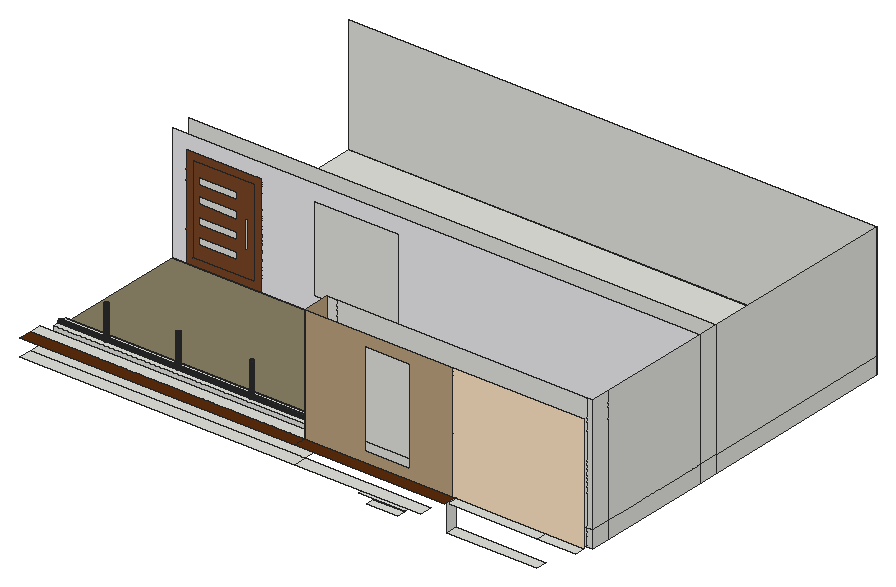
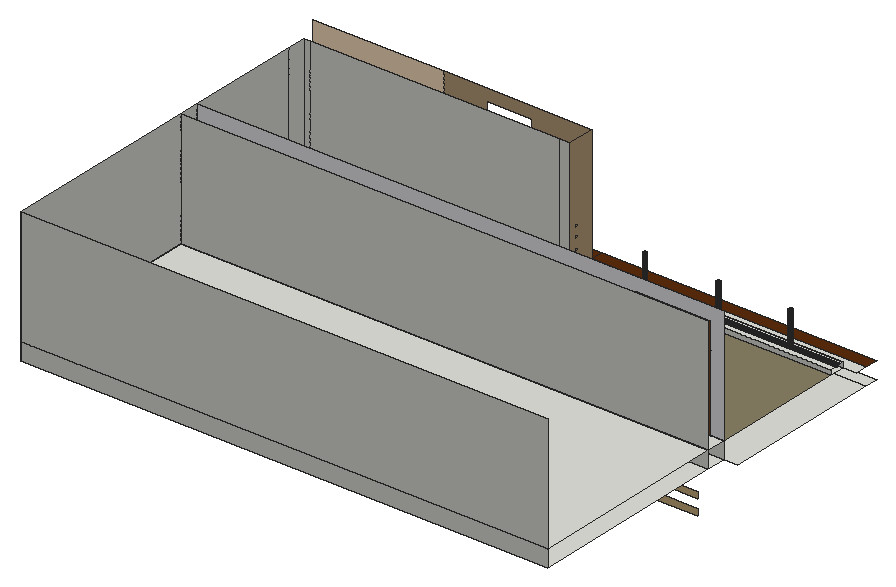
# SketchUp Ruby script. Lengths in inches.
U = 1.inch
M = Sketchup.active_model
def pt(a) = Geom::Point3d.new(a.map { |v| v * U })
def face(e, loops, mat)
  f = e.add_face(loops[0].map { |a| pt(a) })
  loops[1..].each { |l| e.add_face(l.map { |a| pt(a) }).erase! }
  f.material = f.back_material = mat if mat
  f
end
# faces: each face lists its corners as indices into pts; further lists are holes
def faces(e, pts, list, mat = nil) = list.each { |f| face(e, (f[0].is_a?(Array) ? f : [f]).map { |l| l.map { |i| pts[i] } }, mat) }
# xy, xz, yz: faces in a plane at the given z, y or x. An outline is a flat list of corners, or four numbers for a rectangle; further outlines are holes
def ring(l) = l.size == 4 ? [[l[0], l[1]], [l[2], l[1]], [l[2], l[3]], [l[0], l[3]]] : l.each_slice(2).to_a
def flat(e, list, mat, &to3) = list.each { |f| face(e, (f[0].is_a?(Array) ? f : [f]).map { |l| ring(l).map { |u, v| to3.(u, v) } }, mat) }
def xy(e, z, list, mat = nil) = flat(e, list, mat) { |x, y| [x, y, z] }
def xz(e, y, list, mat = nil) = flat(e, list, mat) { |x, z| [x, y, z] }
def yz(e, x, list, mat = nil) = flat(e, list, mat) { |y, z| [x, y, z] }
def lines(e, pts, list) = list.each { |a, b| e.add_line(pt(pts[a]), pt(pts[b])) }
# prism: a flat outline (further loops are holes) pulled along v
def prism(e, loops, v, mat = nil)
  f = face(e, loops, mat); d = Geom::Vector3d.new(v.map { |x| x * U })
  f.pushpull(f.normal.samedirection?(d) ? d.length : -d.length)
end
def box(e, o, s, mat = nil) = prism(e, [[o, [o[0] + s[0], o[1], o[2]], [o[0] + s[0], o[1] + s[1], o[2]], [o[0], o[1] + s[1], o[2]]]], [0, 0, s[2]], mat)
def at(x, y, z, deg = 0) = Geom::Transformation.translation(pt([x, y, z])) * Geom::Transformation.rotation(ORIGIN, Z_AXIS, deg.degrees)
def axes(o, x, y, z) = Geom::Transformation.new([*x, 0, *y, 0, *z, 0, *pt(o).to_a, 1])
def part(name) = M.definitions.add(name)
# library, detail: a bought-in or finely detailed component or shape, given as its bounding box
def library(name, o, s) = part(name).tap { |d| box(d.entities, o, s) }
def detail(e, o, s) = box(e.add_group.entities, o, s)
def put(e, d, t, mat = nil) = e.add_instance(d, t).tap { |i| i.material = mat if mat }
def group(e, t, mat = nil) = e.add_group.tap { |g| g.transformation = t; g.material = mat if mat }.entities
root = M.entities
M.materials.add("[0012_Bisque]").color = [255, 228, 196]
M.materials.add("[0035_Tan]").color = [188, 161, 125]
M.materials.add("[0043_SaddleBrown]").color = [91, 44, 12]
M.materials.add("[Blinds Vertical Pattern]").color = [237, 237, 239]
M.materials.add("[Carpet Pattern Squares Multi]").color = [138, 129, 101]
M.materials.add("[Color M07]").color = [58, 58, 58]
M.materials.add("[Formica Beige]").color = [211, 187, 149]
M.materials.add("[Wood Floor Light]").color = [204, 176, 127]
M.materials.add("[Wood Veneer 01]").color = [120, 70, 37]
xy(root,367.68,[[212.94,538.2,295.68,547.45]],"[Formica Beige]")
xy(root,369.94,[[382.27,385.97,410.625,393.34]])
xy(root,373.6,[[456.39,383.84,537.68,393.34]])
xy(root,376.36,[[375.85,385.97,417.04,393.34]])
xy(root,381.625,[[73.92,382.09,320.99,393.34],[320.99,382.09,434.25,393.34],[73.92,393.34,73.92,538.2,329.72,538.2,329.72,418.04,320.99,418.04,320.99,393.34],[329.72,418.04,560.26,538.2],[85.98,538.2,329.72,556.28],
  [329.72,538.2,560.26,556.28],[85.98,556.28,560.26,737.09]])
xy(root,397.0625,[[456.39,383.84,537.68,393.34],[537.68,383.84,572.32,393.34],[73.92,393.34,320.99,404.34],[[85.98,404.34,320.99,418.04],[128.47,408.87,128.9,408.93,129.31,409.1,129.66,409.36,129.93,409.71,130.1,410.12,130.15,410.56,130.1,410.99,129.93,411.4,129.66,411.75,129.31,412.02,128.9,412.1875,128.47,412.25,128.03,412.1875,127.62,412.02,127.27,411.75,127,411.4,126.84,410.99,126.78,410.56,126.84,410.12,127,409.71,127.27,409.36,127.62,409.1,128.03,408.93],[259.47,408.87,259.9,408.93,260.31,409.1,260.66,409.36,260.93,409.71,261.1,410.12,261.15,410.56,261.1,410.99,260.93,411.4,260.66,411.75,260.31,412.02,259.9,412.1875,259.47,412.25,259.03,412.1875,258.62,412.02,258.27,411.75,258,411.4,257.84,410.99,257.78,410.56,257.84,410.12,258,409.71,258.27,409.36,258.62,409.1,259.03,408.93],[193.34,408.87,193.78,408.93,194.18,409.1,194.53,409.36,194.8,409.71,194.97,410.12,195.03,410.56,194.97,410.99,194.8,411.4,194.53,411.75,194.18,412.02,193.78,412.1875,193.34,412.25,192.9,412.1875,192.5,412.02,192.15,411.75,191.88,411.4,191.71,410.99,191.65,410.56,191.71,410.12,191.88,409.71,192.15,409.36,192.5,409.1,192.9,408.93]],[128.47,408.87,128.03,408.93,127.62,409.1,127.27,409.36,127,409.71,126.84,410.12,126.78,410.56,126.84,410.99,127,411.4,127.27,411.75,127.62,412.02,128.03,412.1875,128.47,412.25,128.9,412.1875,129.31,412.02,129.66,411.75,129.93,411.4,130.1,410.99,130.15,410.56,130.1,410.12,129.93,409.71,129.66,409.36,129.31,409.1,128.9,408.93],
  [193.34,408.87,192.9,408.93,192.5,409.1,192.15,409.36,191.88,409.71,191.71,410.12,191.65,410.56,191.71,410.99,191.88,411.4,192.15,411.75,192.5,412.02,192.9,412.1875,193.34,412.25,193.78,412.1875,194.18,412.02,194.53,411.75,194.8,411.4,194.97,410.99,195.03,410.56,194.97,410.12,194.8,409.71,194.53,409.36,194.18,409.1,193.78,408.93],[259.47,408.87,259.03,408.93,258.62,409.1,258.27,409.36,258,409.71,257.84,410.12,257.78,410.56,257.84,410.99,258,411.4,258.27,411.75,258.62,412.02,259.03,412.1875,259.47,412.25,259.9,412.1875,260.31,412.02,260.66,411.75,260.93,411.4,261.1,410.99,261.15,410.56,261.1,410.12,260.93,409.71,260.66,409.36,260.31,409.1,259.9,408.93],[85.98,538.2,560.26,556.28],[85.98,556.28,560.26,737.09]])
xy(root,397.0625,[[73.92,382.09,320.99,393.34],[320.99,382.09,456.39,393.34]],"[0043_SaddleBrown]")
xy(root,397.0625,[[85.98,418.04,560.26,538.2]],"[Carpet Pattern Squares Multi]")
xy(root,401.4375,[[[85.98,404.34,320.99,418.04],[128.47,408.87,128.03,408.93,127.62,409.1,127.27,409.36,127,409.71,126.84,410.12,126.78,410.56,126.84,410.99,127,411.4,127.27,411.75,127.62,412.02,128.03,412.1875,128.47,412.25,128.9,412.1875,129.31,412.02,129.66,411.75,129.93,411.4,130.1,410.99,130.15,410.56,130.1,410.12,129.93,409.71,129.66,409.36,129.31,409.1,128.9,408.93],[259.47,408.87,259.03,408.93,258.62,409.1,258.27,409.36,258,409.71,257.84,410.12,257.78,410.56,257.84,410.99,258,411.4,258.27,411.75,258.62,412.02,259.03,412.1875,259.47,412.25,259.9,412.1875,260.31,412.02,260.66,411.75,260.93,411.4,261.1,410.99,261.15,410.56,261.1,410.12,260.93,409.71,260.66,409.36,260.31,409.1,259.9,408.93],[193.34,408.87,192.9,408.93,192.5,409.1,192.15,409.36,191.88,409.71,191.71,410.12,191.65,410.56,191.71,410.99,191.88,411.4,192.15,411.75,192.5,412.02,192.9,412.1875,193.34,412.25,193.78,412.1875,194.18,412.02,194.53,411.75,194.8,411.4,194.97,410.99,195.03,410.56,194.97,410.12,194.8,409.71,194.53,409.36,194.18,409.1,193.78,408.93]]])
xz(root,393.34,[[454.48,397.0625,572.32,501.625]],"[0012_Bisque]")
xz(root,393.34,[[[320.99,397.0625,454.48,501.625],[374.52,406.1,415.58,491.35]]],"[0035_Tan]")
xz(root,404.34,[[85.98,397.0625,320.99,401.4375]])
xz(root,418.04,[[320.99,381.625,329.72,397.0625],[329.72,381.625,554.62,397.0625],[554.62,381.625,560.26,397.0625],[85.98,397.0625,320.99,401.4375],[320.99,397.0625,329.72,501.625],
  [329.72,397.0625,554.62,501.625],[554.62,397.0625,560.26,501.625]])
xz(root,538.2,[[85.98,381.625,560.26,397.0625]])
xz(root,538.2,[[[85.98,397.0625,97.73,397.0625,97.73,489,166.42,489,166.42,397.0625,560.26,397.0625,560.26,501.625,85.98,501.625],[213.51,411.53,289.58,487.59]]],"[Blinds Vertical Pattern]")
xz(root,538.2,[[109.29,327.9,145.13,333.78],[109.29,341.71,145.13,347.59]],"[Wood Floor Light]")
xz(root,538.2,[[[97.73,397.0625,166.42,489],[104.37,403.7,159.78,482.36]],[[104.37,403.7,159.78,482.36],[109.29,463.85,144.04,470.66],[109.29,448.48,144.04,455.29],[109.29,431.66,144.04,438.48],[109.29,415.48,144.04,422.29],[150.7,427.01,154.02,451.83]]],"[Wood Veneer 01]")
xz(root,556.28,[[85.98,381.625,560.26,397.0625],[85.98,397.0625,560.26,501.625]])
xz(root,737.09,[[85.98,381.625,560.26,397.0625],[85.98,397.0625,560.26,501.625]])
yz(root,320.99,[[404.34,397.0625,404.34,401.4375,409.49,401.4375,409.6,401.18,409.875,400.82,410.24,400.54,410.66,400.36,411.11,400.3,411.57,400.36,411.99,400.54,412.35,400.82,412.63,401.18,412.73,401.4375,418.04,401.4375,418.04,397.0625],[411.11,400.3,411.57,400.36,411.99,400.54,412.35,400.82,412.63,401.18,412.73,401.4375,409.49,401.4375,409.6,401.18,409.875,400.82,410.24,400.54,410.66,400.36]])
yz(root,320.99,[[[393.34,397.0625,393.34,501.625,418.04,501.625,418.04,401.4375,412.73,401.4375,412.8,401.6,412.86,402.05,412.8,402.51,412.63,402.93,412.35,403.29,411.99,403.57,411.57,403.75,411.11,403.8,410.66,403.75,410.24,403.57,409.875,403.29,409.6,402.93,409.42,402.51,409.36,402.05,409.42,401.6,409.49,401.4375,404.34,401.4375,404.34,397.0625],[411.11,410.55,411.57,410.61,411.99,410.79,412.35,411.07,412.63,411.43,412.8,411.85,412.86,412.3,412.8,412.76,412.63,413.18,412.35,413.54,411.99,413.82,411.57,414,411.11,414.05,410.66,414,410.24,413.82,409.875,413.54,409.6,413.18,409.42,412.76,409.36,412.3,409.42,411.85,409.6,411.43,409.875,411.07,410.24,410.79,410.66,410.61],[411.11,420.8,411.57,420.86,411.99,421.04,412.35,421.32,412.63,421.68,412.8,422.1,412.86,422.55,412.8,423.01,412.63,423.43,412.35,423.79,411.99,424.07,411.57,424.25,411.11,424.3,410.66,424.25,410.24,424.07,409.875,423.79,409.6,423.43,409.42,423.01,409.36,422.55,409.42,422.1,409.6,421.68,409.875,421.32,410.24,421.04,410.66,420.86],[411.11,429.99,411.57,430.05,411.99,430.23,412.35,430.51,412.63,430.87,412.8,431.29,412.86,431.74,412.8,432.2,412.63,432.62,412.35,432.98,411.99,433.26,411.57,433.43,411.11,433.49,410.66,433.43,410.24,433.26,409.875,432.98,409.6,432.62,409.42,432.2,409.36,431.74,409.42,431.29,409.6,430.87,409.875,430.51,410.24,430.23,410.66,430.05]]],"[0035_Tan]")
yz(root,456.39,[[383.84,373.6,393.34,397.0625]])
yz(root,560.26,[[418.04,381.625,434.85,397.0625],[434.85,381.625,538.2,397.0625],[538.2,381.625,556.28,397.0625],[556.28,381.625,737.09,397.0625],[418.04,397.0625,434.85,501.625],
  [434.85,397.0625,538.2,501.625],[538.2,397.0625,556.28,501.625],[556.28,397.0625,737.09,501.625]])
p = [[127.62,409.1,397.0625],[128.03,408.93,397.0625],[128.03,408.93,401.4375],[127.62,409.1,401.4375],[128.47,408.87,397.0625],[128.47,408.87,401.4375],
  [128.9,408.93,397.0625],[128.9,408.93,401.4375],[129.31,409.1,397.0625],[129.31,409.1,401.4375],[192.5,409.1,397.0625],[192.9,408.93,397.0625],
  [192.9,408.93,401.4375],[192.5,409.1,401.4375],[193.34,408.87,397.0625],[193.34,408.87,401.4375],[193.78,408.93,397.0625],[193.78,408.93,401.4375],
  [194.18,409.1,397.0625],[194.18,409.1,401.4375],[258.62,409.1,397.0625],[259.03,408.93,397.0625],[259.03,408.93,401.4375],[258.62,409.1,401.4375],
  [259.47,408.87,397.0625],[259.47,408.87,401.4375],[259.9,408.93,397.0625],[259.9,408.93,401.4375],[260.31,409.1,397.0625],[260.31,409.1,401.4375],
  [127.27,409.36,397.0625],[127.27,409.36,401.4375],[129.66,409.36,397.0625],[129.66,409.36,401.4375],[192.15,409.36,397.0625],[192.15,409.36,401.4375],
  [194.53,409.36,397.0625],[194.53,409.36,401.4375],[258.27,409.36,397.0625],[258.27,409.36,401.4375],[260.66,409.36,397.0625],[260.66,409.36,401.4375],
  [127,409.71,397.0625],[127,409.71,401.4375],[129.93,409.71,397.0625],[129.93,409.71,401.4375],[191.88,409.71,397.0625],[191.88,409.71,401.4375],
  [194.8,409.71,397.0625],[194.8,409.71,401.4375],[258,409.71,397.0625],[258,409.71,401.4375],[260.93,409.71,397.0625],[260.93,409.71,401.4375],
  [126.84,410.12,397.0625],[126.84,410.12,401.4375],[130.1,410.12,397.0625],[130.1,410.12,401.4375],[191.71,410.12,397.0625],[191.71,410.12,401.4375],
  [194.97,410.12,397.0625],[194.97,410.12,401.4375],[257.84,410.12,397.0625],[257.84,410.12,401.4375],[261.1,410.12,397.0625],[261.1,410.12,401.4375],
  [130.15,410.56,397.0625],[130.15,410.56,401.4375],[191.65,410.56,397.0625],[191.65,410.56,401.4375],[195.03,410.56,397.0625],[195.03,410.56,401.4375],
  [257.78,410.56,397.0625],[257.78,410.56,401.4375],[261.15,410.56,397.0625],[261.15,410.56,401.4375],[130.1,410.99,397.0625],[130.1,410.99,401.4375],
  [191.71,410.99,397.0625],[191.71,410.99,401.4375],[194.97,410.99,397.0625],[194.97,410.99,401.4375],[257.84,410.99,397.0625],[257.84,410.99,401.4375],
  [261.1,410.99,397.0625],[261.1,410.99,401.4375],[127,411.4,397.0625],[126.84,410.99,397.0625],[126.84,410.99,401.4375],[127,411.4,401.4375],
  [129.93,411.4,397.0625],[129.93,411.4,401.4375],[191.88,411.4,397.0625],[191.88,411.4,401.4375],[194.8,411.4,397.0625],[194.8,411.4,401.4375],
  [258,411.4,397.0625],[258,411.4,401.4375],[260.93,411.4,397.0625],[260.93,411.4,401.4375],[127.27,411.75,397.0625],[127.27,411.75,401.4375],
  [129.66,411.75,397.0625],[129.66,411.75,401.4375],[192.15,411.75,397.0625],[192.15,411.75,401.4375],[194.53,411.75,397.0625],[194.53,411.75,401.4375],
  [258.27,411.75,397.0625],[258.27,411.75,401.4375],[260.66,411.75,397.0625],[260.66,411.75,401.4375],[127.62,412.02,397.0625],[127.62,412.02,401.4375],
  [129.31,412.02,397.0625],[129.31,412.02,401.4375],[192.5,412.02,397.0625],[192.5,412.02,401.4375],[194.18,412.02,397.0625],[194.18,412.02,401.4375],
  [258.62,412.02,397.0625],[258.62,412.02,401.4375],[260.31,412.02,397.0625],[260.31,412.02,401.4375],[128.03,412.1875,397.0625],[128.03,412.1875,401.4375],
  [128.9,412.1875,397.0625],[128.9,412.1875,401.4375],[192.9,412.1875,397.0625],[192.9,412.1875,401.4375],[193.78,412.1875,397.0625],[193.78,412.1875,401.4375],
  [259.03,412.1875,397.0625],[259.03,412.1875,401.4375],[259.9,412.1875,397.0625],[259.9,412.1875,401.4375],[128.47,412.25,397.0625],[128.47,412.25,401.4375],
  [193.34,412.25,397.0625],[193.34,412.25,401.4375],[259.47,412.25,397.0625],[259.47,412.25,401.4375],[85.98,410.66,400.36],[85.98,411.11,400.3],
  [320.99,411.11,400.3],[320.99,410.66,400.36],[85.98,411.57,400.36],[320.99,411.57,400.36],[85.98,410.24,400.54],[320.99,410.24,400.54],
  [85.98,411.99,400.54],[320.99,411.99,400.54],[85.98,409.875,400.82],[320.99,409.875,400.82],[85.98,412.35,400.82],[320.99,412.35,400.82],
  [85.98,409.6,401.18],[320.99,409.6,401.18],[85.98,412.63,401.18],[320.99,412.63,401.18],[85.98,409.49,401.4375],[320.99,409.49,401.4375],
  [320.99,409.42,401.6],[85.98,409.42,401.6],[85.98,412.73,401.4375],[85.98,412.8,401.6],[320.99,412.8,401.6],[320.99,412.73,401.4375],
  [127.62,409.1,431.75],[128.03,408.93,431.75],[128.47,408.87,431.75],[128.9,408.93,431.75],[129.31,409.1,431.75],[192.5,409.1,431.4375],
  [192.9,408.93,431.4375],[193.34,408.87,431.4375],[193.78,408.93,431.4375],[194.18,409.1,431.4375],[258.62,409.1,431.5625],[259.03,408.93,431.5625],
  [259.47,408.87,431.5625],[259.9,408.93,431.5625],[260.31,409.1,431.5625],[127.27,409.36,431.75],[129.66,409.36,431.75],[192.15,409.36,431.4375],
  [194.53,409.36,431.4375],[258.27,409.36,431.5625],[260.66,409.36,431.5625],[127,409.71,431.75],[129.93,409.71,431.75],[191.88,409.71,431.4375],
  [194.8,409.71,431.4375],[258,409.71,431.5625],[260.93,409.71,431.5625],[126.84,410.12,431.75],[130.1,410.12,431.75],[191.71,410.12,431.4375],
  [194.97,410.12,431.4375],[257.84,410.12,431.5625],[261.1,410.12,431.5625],[126.78,410.56,431.75],[126.78,410.56,401.4375],[130.15,410.56,431.75],
  [191.65,410.56,431.4375],[195.03,410.56,431.4375],[257.78,410.56,431.5625],[261.15,410.56,431.5625],[126.84,410.99,431.75],[130.1,410.99,431.75],
  [191.71,410.99,431.4375],[194.97,410.99,431.4375],[257.84,410.99,431.5625],[261.1,410.99,431.5625],[127,411.4,431.75],[129.93,411.4,431.75],
  [191.88,411.4,431.4375],[194.8,411.4,431.4375],[258,411.4,431.5625],[260.93,411.4,431.5625],[127.27,411.75,431.75],[129.66,411.75,431.75],
  [192.15,411.75,431.4375],[194.53,411.75,431.4375],[258.27,411.75,431.5625],[260.66,411.75,431.5625],[127.62,412.02,431.75],[129.31,412.02,431.75],
  [192.5,412.02,431.4375],[194.18,412.02,431.4375],[258.62,412.02,431.5625],[260.31,412.02,431.5625],[128.03,412.1875,431.75],[128.9,412.1875,431.75],
  [192.9,412.1875,431.4375],[193.78,412.1875,431.4375],[259.03,412.1875,431.5625],[259.9,412.1875,431.5625],[128.47,412.25,431.75],[193.34,412.25,431.4375],
  [259.47,412.25,431.5625],[85.98,409.36,402.05],[320.99,409.36,402.05],[85.98,412.86,402.05],[320.99,412.86,402.05],[85.98,409.42,402.51],
  [320.99,409.42,402.51],[85.98,412.8,402.51],[320.99,412.8,402.51],[85.98,409.6,402.93],[320.99,409.6,402.93],[85.98,412.63,402.93],
  [320.99,412.63,402.93],[85.98,409.875,403.29],[320.99,409.875,403.29],[85.98,412.35,403.29],[320.99,412.35,403.29],[85.98,410.24,403.57],
  [320.99,410.24,403.57],[85.98,411.99,403.57],[320.99,411.99,403.57],[85.98,410.66,403.75],[320.99,410.66,403.75],[85.98,411.57,403.75],
  [320.99,411.57,403.75],[85.98,411.11,403.8],[320.99,411.11,403.8]]
faces(root,p,[[0,1,2,3],[1,4,5,2],[4,6,7,5],[6,8,9,7],[10,11,12,13],[11,14,15,12],[14,16,17,15],[16,18,19,17],
  [20,21,22,23],[21,24,25,22],[24,26,27,25],[26,28,29,27],[30,0,3,31],[8,32,33,9],[34,10,13,35],[18,36,37,19],
  [38,20,23,39],[28,40,41,29],[42,30,31,43],[32,44,45,33],[46,34,35,47],[36,48,49,37],[50,38,39,51],[40,52,53,41],
  [54,42,43,55],[44,56,57,45],[58,46,47,59],[48,60,61,49],[62,50,51,63],[52,64,65,53],[56,66,67,57],[68,58,59,69],
  [60,70,71,61],[72,62,63,73],[64,74,75,65],[66,76,77,67],[78,68,69,79],[70,80,81,71],[82,72,73,83],[74,84,85,75],
  [86,87,88,89],[76,90,91,77],[92,78,79,93],[80,94,95,81],[96,82,83,97],[84,98,99,85],[100,86,89,101],[90,102,103,91],
  [104,92,93,105],[94,106,107,95],[108,96,97,109],[98,110,111,99],[112,100,101,113],[102,114,115,103],[116,104,105,117],[106,118,119,107],
  [120,108,109,121],[110,122,123,111],[124,112,113,125],[114,126,127,115],[128,116,117,129],[118,130,131,119],[132,120,121,133],[122,134,135,123],
  [136,124,125,137],[126,136,137,127],[138,128,129,139],[130,138,139,131],[140,132,133,141],[134,140,141,135]])
faces(root,p,[[142,143,144,145],[143,146,147,144],[148,142,145,149],[146,150,151,147],[152,148,149,153],[150,154,155,151],[156,152,153,157],[154,158,159,155],
  [160,156,157,161,162,163],[164,165,166,167,159,158],[168,3,2,169],[169,2,5,170],[170,5,7,171],[171,7,9,172],[173,13,12,174],[174,12,15,175],
  [175,15,17,176],[176,17,19,177],[178,23,22,179],[179,22,25,180],[180,25,27,181],[181,27,29,182],[183,31,3,168],[172,9,33,184],
  [185,35,13,173],[177,19,37,186],[187,39,23,178],[182,29,41,188],[189,43,31,183],[184,33,45,190],[191,47,35,185],[186,37,49,192],
  [193,51,39,187],[188,41,53,194],[195,55,43,189],[190,45,57,196],[197,59,47,191],[192,49,61,198],[199,63,51,193],[194,53,65,200],
  [201,202,55,195],[196,57,67,203],[204,69,59,197],[198,61,71,205],[206,73,63,199],[200,65,75,207],[208,88,202,201],[203,67,77,209],
  [210,79,69,204],[205,71,81,211],[212,83,73,206],[207,75,85,213],[214,89,88,208],[209,77,91,215],[216,93,79,210],[211,81,95,217],
  [218,97,83,212],[213,85,99,219],[220,101,89,214],[215,91,103,221],[222,105,93,216],[217,95,107,223],[224,109,97,218],[219,99,111,225],
  [226,113,101,220],[221,103,115,227],[228,117,105,222],[223,107,119,229],[230,121,109,224],[225,111,123,231],[232,125,113,226],[227,115,127,233],
  [234,129,117,228],[229,119,131,235],[236,133,121,230],[231,123,135,237],[238,137,125,232],[233,127,137,238],[239,139,129,234],[235,131,139,239],
  [240,141,133,236],[237,135,141,240],[241,163,162,242],[165,243,244,166],[245,241,242,246],[243,247,248,244],[249,245,246,250],[247,251,252,248],
  [253,249,250,254],[251,255,256,252],[257,253,254,258],[255,259,260,256],[261,257,258,262],[259,263,264,260],[265,261,262,266],[263,265,266,264]],"[Color M07]")
